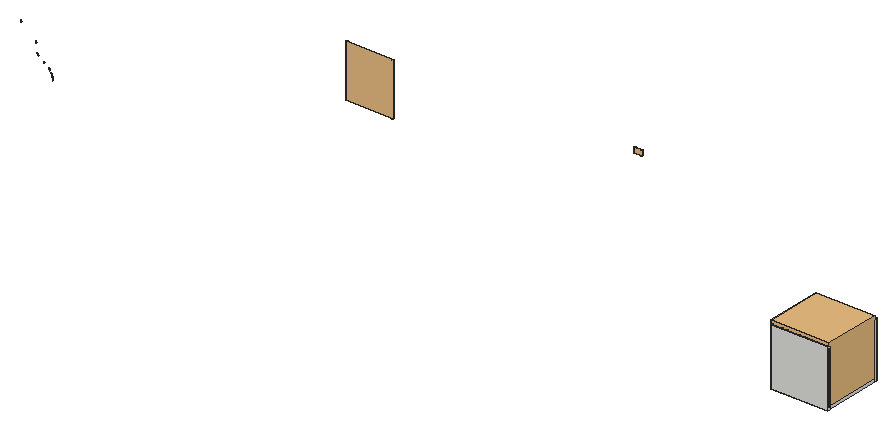
# SketchUp Ruby script. Lengths in inches.
U = 1.inch
M = Sketchup.active_model
def pt(a) = Geom::Point3d.new(a.map { |v| v * U })
def face(e, loops, mat)
  f = e.add_face(loops[0].map { |a| pt(a) })
  loops[1..].each { |l| e.add_face(l.map { |a| pt(a) }).erase! }
  f.material = f.back_material = mat if mat
  f
end
# faces: each face lists its corners as indices into pts; further lists are holes
def faces(e, pts, list, mat = nil) = list.each { |f| face(e, (f[0].is_a?(Array) ? f : [f]).map { |l| l.map { |i| pts[i] } }, mat) }
# xy, xz, yz: faces in a plane at the given z, y or x. An outline is a flat list of corners, or four numbers for a rectangle; further outlines are holes
def ring(l) = l.size == 4 ? [[l[0], l[1]], [l[2], l[1]], [l[2], l[3]], [l[0], l[3]]] : l.each_slice(2).to_a
def flat(e, list, mat, &to3) = list.each { |f| face(e, (f[0].is_a?(Array) ? f : [f]).map { |l| ring(l).map { |u, v| to3.(u, v) } }, mat) }
def xy(e, z, list, mat = nil) = flat(e, list, mat) { |x, y| [x, y, z] }
def xz(e, y, list, mat = nil) = flat(e, list, mat) { |x, z| [x, y, z] }
def yz(e, x, list, mat = nil) = flat(e, list, mat) { |y, z| [x, y, z] }
def lines(e, pts, list) = list.each { |a, b| e.add_line(pt(pts[a]), pt(pts[b])) }
# prism: a flat outline (further loops are holes) pulled along v
def prism(e, loops, v, mat = nil)
  f = face(e, loops, mat); d = Geom::Vector3d.new(v.map { |x| x * U })
  f.pushpull(f.normal.samedirection?(d) ? d.length : -d.length)
end
def box(e, o, s, mat = nil) = prism(e, [[o, [o[0] + s[0], o[1], o[2]], [o[0] + s[0], o[1] + s[1], o[2]], [o[0], o[1] + s[1], o[2]]]], [0, 0, s[2]], mat)
def at(x, y, z, deg = 0) = Geom::Transformation.translation(pt([x, y, z])) * Geom::Transformation.rotation(ORIGIN, Z_AXIS, deg.degrees)
def axes(o, x, y, z) = Geom::Transformation.new([*x, 0, *y, 0, *z, 0, *pt(o).to_a, 1])
def part(name) = M.definitions.add(name)
# library, detail: a bought-in or finely detailed component or shape, given as its bounding box
def library(name, o, s) = part(name).tap { |d| box(d.entities, o, s) }
def detail(e, o, s) = box(e.add_group.entities, o, s)
def put(e, d, t, mat = nil) = e.add_instance(d, t).tap { |i| i.material = mat if mat }
def group(e, t, mat = nil) = e.add_group.tap { |g| g.transformation = t; g.material = mat if mat }.entities
root = M.entities
M.materials.add("Generic\#1").color = [212, 210, 207]
M.materials["Generic\#1"].alpha = 0.64
M.materials.add("[Color_C17]").color = [102, 61, 19]
M.materials.add("[Color_D04]").color = [226, 212, 151]
M.materials.add("[Metal Corrugated Shiny]").color = [126, 126, 126]
M.materials.add("[Translucent Glass Gray]1").color = [186, 186, 186]
M.materials["[Translucent Glass Gray]1"].alpha = 0.5
M.materials.add("[Translucent Glass Gray]2").color = [128, 128, 128]
M.materials["[Translucent Glass Gray]2"].alpha = 0.5
M.materials.add("guide_book_pages_650").color = [228, 220, 176]
M.materials.add("wall texture").color = [149, 150, 148]
c1 = library("bed",[8.45,-2.17,-0.02],[100.66,82.09,31.1])
c2 = part("Grupo\#10")
prism(c2.entities,[[[0.34,1.25,0],[0.5,1.32,0],[0.67,1.34,0],[0.85,1.32,0],[1.01,1.25,0],[1.15,1.15,0],[1.25,1.01,0],[1.32,0.85,0],[1.34,0.67,0],[1.32,0.5,0],[1.25,0.34,0],[1.15,0.2,0],[1.01,0.09,0],[0.85,0.02,0],[0.67,0,0],[0.5,0.02,0],[0.34,0.09,0],[0.2,0.2,0],[0.09,0.34,0],[0.02,0.5,0],[0,0.67,0],[0.02,0.85,0],[0.09,1.01,0],[0.2,1.15,0]]],[0,0,192.91])
c3 = part("Grupo\#1")
put(c3.entities,c2,axes([8.8125,2.875,0.56],[0.0689,0,0],[0,0.06833,0.00887],[0,-0.00887,0.06833]))
put(c3.entities,c2,axes([9.19,1.3125,0.58],[0.06879,0.00048,0.00394],[0,0.0684,-0.00828],[-0.00397,0.00826,0.06829]))
put(c3.entities,c2,axes([8.9,0.97,1.35],[0.0689,0,0],[0,0.06788,-0.01185],[0,0.01185,0.06788]))
put(c3.entities,c2,axes([9.375,1.96,0.37],[0.06868,0,0.00553],[0,0.0689,0],[-0.00553,0,0.06868]))
put(c3.entities,c2,axes([7.76,2.02,1.22],[0.06788,0,-0.01185],[0,0.0689,0],[0.01185,0,0.06788]))
g1 = group(c3.entities,at(6.375,-0.82,0))
detail(g1,[0,0,0],[4.31,4.31,6.9375])
c4 = part("Difusor aromático\#1")
put(c4.entities,c3,at(-1.02,1.61,-0.92),"[Translucent Glass Gray]2")
c5 = part("Book\#1")
xy(c5.entities,0,[[0,0,199.1,147.6]],"[Color_C17]")
xy(c5.entities,1.64,[[0,0,3.4,147.6],[195.7,0,199.1,147.6]],"[Color_C17]")
xz(c5.entities,0,[[0,0,199.1,1.64]],"[Color_C17]")
xz(c5.entities,0,[[3.4,1.64,195.7,1.64,193.74,6.22,190.64,6.23,187.55,6.32,184.47,6.49,181.39,6.75,178.34,7.1,175.31,7.53,172.3,8.04,166.83,9.33,161.3,10.51,155.73,11.57,150.11,12.51,144.46,13.33,138.77,14.04,133.05,14.62,127.79,14.85,122.53,14.58,117.37,13.8125,112.4,12.57,107.72,10.87,103.41,8.74,99.55,6.22,95.6875,9.67,91.38,12.58,86.7,14.92,81.73,16.62,76.57,17.67,71.3125,18.04,66.05,17.73,60.33,16.93,54.64,15.96,48.99,14.84,43.37,13.55,37.8,12.1,32.27,10.48,26.8,8.71,23.79,8.01,20.76,7.42,17.71,6.95,14.64,6.59,11.55,6.35,8.46,6.23,5.37,6.22]],"[Color_D04]")
xz(c5.entities,147.6,[[0,0,199.1,1.64]],"[Color_C17]")
xz(c5.entities,147.6,[[3.4,1.64,5.37,6.22,8.46,6.23,11.55,6.35,14.64,6.59,17.71,6.95,20.76,7.42,23.79,8.01,26.8,8.71,32.27,10.48,37.8,12.1,43.37,13.55,48.99,14.84,54.64,15.96,60.33,16.93,66.05,17.73,71.3125,18.04,76.57,17.67,81.73,16.62,86.7,14.92,91.38,12.58,95.6875,9.67,99.55,6.22,103.41,8.74,107.72,10.87,112.4,12.57,117.37,13.8125,122.53,14.58,127.79,14.85,133.05,14.62,138.77,14.04,144.46,13.33,150.11,12.51,155.73,11.57,161.3,10.51,166.83,9.33,172.3,8.04,175.31,7.53,178.34,7.1,181.39,6.75,184.47,6.49,187.55,6.32,190.64,6.23,193.74,6.22,195.7,1.64]],"[Color_D04]")
yz(c5.entities,0,[[0,0,147.6,1.64]],"[Color_C17]")
yz(c5.entities,199.1,[[0,0,147.6,1.64]],"[Color_C17]")
p = [[3.4,0,1.64],[5.37,0,6.22],[5.37,147.6,6.22],[3.4,147.6,1.64],[193.74,0,6.22],[195.7,0,1.64],
  [195.7,147.6,1.64],[193.74,147.6,6.22],[8.46,0,6.23],[8.46,147.6,6.23],[11.55,0,6.35],[11.55,147.6,6.35],
  [95.6875,0,9.67],[99.55,0,6.22],[99.55,147.6,6.22],[95.6875,147.6,9.67],[103.41,0,8.74],[103.41,147.6,8.74],
  [187.55,0,6.32],[190.64,0,6.23],[190.64,147.6,6.23],[187.55,147.6,6.32],[184.47,0,6.49],[184.47,147.6,6.49],
  [14.64,0,6.59],[14.64,147.6,6.59],[181.39,0,6.75],[181.39,147.6,6.75],[17.71,0,6.95],[17.71,147.6,6.95],
  [178.34,0,7.1],[178.34,147.6,7.1],[20.76,0,7.42],[20.76,147.6,7.42],[175.31,0,7.53],[175.31,147.6,7.53],
  [23.79,0,8.01],[23.79,147.6,8.01],[172.3,0,8.04],[172.3,147.6,8.04],[26.8,0,8.71],[26.8,147.6,8.71],
  [166.83,0,9.33],[166.83,147.6,9.33],[32.27,0,10.48],[32.27,147.6,10.48],[107.72,0,10.87],[107.72,147.6,10.87],
  [161.3,0,10.51],[161.3,147.6,10.51],[91.38,0,12.58],[91.38,147.6,12.58],[37.8,0,12.1],[37.8,147.6,12.1],
  [155.73,0,11.57],[155.73,147.6,11.57],[112.4,0,12.57],[112.4,147.6,12.57],[150.11,0,12.51],[150.11,147.6,12.51],
  [43.37,0,13.55],[43.37,147.6,13.55],[144.46,0,13.33],[144.46,147.6,13.33],[86.7,0,14.92],[86.7,147.6,14.92],
  [117.37,0,13.8125],[117.37,147.6,13.8125],[138.77,0,14.04],[138.77,147.6,14.04],[48.99,0,14.84],[48.99,147.6,14.84],
  [122.53,0,14.58],[122.53,147.6,14.58],[133.05,0,14.62],[133.05,147.6,14.62],[127.79,0,14.85],[127.79,147.6,14.85],
  [54.64,0,15.96],[54.64,147.6,15.96],[81.73,0,16.62],[81.73,147.6,16.62],[60.33,0,16.93],[60.33,147.6,16.93],
  [76.57,0,17.67],[76.57,147.6,17.67],[66.05,0,17.73],[66.05,147.6,17.73],[71.3125,0,18.04],[71.3125,147.6,18.04]]
faces(c5.entities,p,[[0,1,2,3],[4,5,6,7],[1,8,9,2],[8,10,11,9],[12,13,14,15],[13,16,17,14],[18,19,20,21],[19,4,7,20],
  [22,18,21,23],[10,24,25,11],[26,22,23,27],[24,28,29,25],[30,26,27,31],[28,32,33,29],[34,30,31,35],[32,36,37,33],
  [38,34,35,39],[36,40,41,37],[42,38,39,43],[40,44,45,41],[16,46,47,17],[48,42,43,49],[50,12,15,51],[44,52,53,45],
  [54,48,49,55],[46,56,57,47],[58,54,55,59],[52,60,61,53],[62,58,59,63],[64,50,51,65],[56,66,67,57],[68,62,63,69],
  [60,70,71,61],[66,72,73,67],[74,68,69,75],[72,76,77,73],[76,74,75,77],[70,78,79,71],[80,64,65,81],[78,82,83,79],
  [84,80,81,85],[82,86,87,83],[86,88,89,87],[88,84,85,89]],"guide_book_pages_650")
c6 = library("Glasses\#1",[0,0,0],[79.32,78.74,17.6])
c7 = library("Group\#5",[0,0,0],[21.15,0.01,14.26])
c8 = library("Group\#8",[0,0,0],[102.14,0.5,111.36])
c9 = library("Group\#17",[0,0,0],[28.72,28.74,77])
c10 = part("Square rod")
xy(c10.entities,-0.04,[[0.04,0.04,0.36,0.36]])
xy(c10.entities,0,[[[0,0,0.39,0.39],[0.04,0.04,0.36,0.36]]])
xy(c10.entities,19.69,[[0,0,0.39,0.39]])
xz(c10.entities,0,[[0,0,0.39,19.69]])
xz(c10.entities,0.04,[[0.04,-0.04,0.36,0]])
xz(c10.entities,0.36,[[0.04,-0.04,0.36,0]])
xz(c10.entities,0.39,[[0,0,0.39,19.69]])
yz(c10.entities,0,[[0,0,0.39,19.69]])
yz(c10.entities,0.04,[[0.04,-0.04,0.36,0]])
yz(c10.entities,0.36,[[0.04,-0.04,0.36,0]])
yz(c10.entities,0.39,[[0,0,0.39,19.69]])
c11 = part("Group\#626")
box(c11.entities,[0,0,0],[0.39,18.9,0.39])
c12 = part("Group\#630")
box(c12.entities,[0,0,0],[18.9,0.39,0.39])
c13 = library("Group\#635",[0,0,0],[3.14,3.14,10.11])
c14 = library("Group\#634",[0,0,0],[7.05,7.05,10.1])
c15 = library("Group\#633",[0,0,0],[47.27,36.83,57.22])
c16 = library("Group\#632",[0,0,0],[63.43,39.67,4.76])
c17 = library("Group\#639",[0,0,0],[29.35,22.46,29.82])
xz(root,68.94,[[68.26,0,67.897,2.998,67.579,4.474,67.288,5.822,68.136,6.149,68.144,6.152,68.135,6.15,67.632,6.075,67.231,6.044,66.358,8.824,67.116,7.869,68.125,6.184,67.294,8.831,66.128,11.616,64.712,14.283,63.056,16.809,61.45,18.827,61.176,19.172,59.596,20.821,60.055,20.229,61.45,18.827,63.056,16.809,64.712,14.283,66.128,11.616,67.294,8.831,68.125,6.184,68.135,6.15,68.136,6.149,68.198,5.95,68.516,4.474,68.835,2.998,69.197,0],[61.45,18.827,60.055,20.229,59.596,20.821,61.176,19.172],[50.479,26.777,50.392,26.818,50.718,27.105],[50.718,27.105,49.015,27.904,48.649,28.08,48.921,27.989],[38.749,35.828,38.683,35.912,38.746,35.834],
  [38.683,35.912,38.208,36.506,38.149,36.599],[38.149,36.599,37.535,37.389,36.522,39.088,35.726,40.898,35.718,40.926,36.714,38.871],[32.979,59.945,32.975,59.997,32.405,62.383,32.196,62.884,32.966,61.774,33.882,59.994,33.365,59.95],[1.729,87.284,1.661,87.435,0.638,89.676,0,90.727,0.145,90.599,1.465,89.094,2.576,87.429,2.068,87.327]])
# 1073 loose lines left out
detail(root,[485.1,319.58,0.05],[101.58,0.05,110.82])
detail(root,[1634.04,3.5,0],[124,120,126])
put(root,c1,axes([1701.17,19.22,6.01],[0,0.79,0],[-0.79,0,0],[0,0,0.79]))
put(root,c4,axes([1650.16,104.91,26],[0.29449,-0.03616,0],[0.03616,0.29449,0],[0,0,0.2967]))
put(root,c5,axes([1659.12,112.75,21.39],[0.01748,-0.03819,0],[0.03819,0.01748,0],[0,0,0.042]))
put(root,c6,axes([1660.36,111.62,22.1875],[0.01391,-0.0393,-0.00511],[0.03953,0.01414,-0.00114],[0.00279,-0.00443,0.04167]))
g2 = group(root,at(1758.04,3.5,0,90))
xy(g2,0,[[0,0,120,120]])
xy(g2,6,[[0,0,120,120]],"Generic\#1")
xz(g2,0,[[0,0,120,6]])
xz(g2,120,[[0,0,120,6]])
yz(g2,0,[[0,0,120,6]])
yz(g2,120,[[0,0,120,6]])
g3 = group(root,at(1758.04,127.5,0,180))
xy(g3,0,[[0,0,120,4]])
xy(g3,120,[[0,0,120,4]])
xz(g3,0,[[0,0,120,120]])
xz(g3,4,[[0,0,120,120]],"wall texture")
yz(g3,0,[[0,0,4,120]])
yz(g3,120,[[0,0,4,120]])
put(root,c7,axes([968.64,475.68,1.17],[0.86,0,0],[0,0.86,0],[0,0,0.86]))
g4 = group(root,at(1638.04,0,6))
xy(g4,-6,[[0,0,120,4]])
xy(g4,114,[[0,0,120,4]])
xz(g4,0,[[0,-6,120,114]])
xz(g4,4,[[118.939,5.841,118.938,5.843,118.947,5.844]])
yz(g4,0,[[0,-6,4,114]])
yz(g4,120,[[0,-6,4,114]])
# 341 loose lines left out
detail(g4,[0.02,2,0.03],[120,1.5,114])
put(g4,c8,axes([17.86,3.6875,0],[1,0,0],[0,1,0],[0,0,0.95]))
put(root,c9,axes([1649.82,10.52,79.19],[0.53,0,0],[0,0.53,0],[0,0,0.53]))
put(root,c9,axes([1644.52,108.27,79.19],[0.53,0,0],[0,0.53,0],[0,0,0.53]))
g5 = group(root,at(1640.91,8.49,21.39))
xy(g5,0,[[[0,0,19.291,18.898],[0.394,0.394,18.898,18.504]],[0.394,0.394,18.898,18.504]])
xy(g5,1.581,[[0,0,18.898,0.197],[0,18.701,18.898,18.898]])
xy(g5,2.172,[[0,0,18.898,0.197],[0,18.701,18.898,18.898]])
xy(g5,3.917,[[0,0,19.291,0,19.291,7.874,18.898,7.874,18.898,0.394,0.394,0.394,0.394,18.504,18.898,18.504,18.898,11.024,19.291,11.024,19.291,18.898,0,18.898]])
xz(g5,0,[[0,0,19.291,0,19.291,3.917,0,3.917,0,2.172,18.898,2.172,18.898,1.581,0,1.581]])
xz(g5,0.197,[[0,1.581,18.898,2.172]])
xz(g5,0.394,[[0.394,0,18.898,3.917]])
xz(g5,18.504,[[0.394,0,18.898,3.917]])
xz(g5,18.701,[[0,1.581,18.898,2.172]])
xz(g5,18.898,[[0,0,0,1.581,18.898,1.581,18.898,2.172,0,2.172,0,3.917,19.291,3.917,19.291,0]])
yz(g5,0,[[0,0,0,1.581,0.197,1.581,0.197,2.172,0,2.172,0,3.917,18.898,3.917,18.898,2.172,18.701,2.172,18.701,1.581,18.898,1.581,18.898,0]])
yz(g5,0.394,[[0.394,0,18.504,3.917]])
yz(g5,18.898,[[0.394,0,0.394,3.917,7.874,3.917,7.874,3.937,7.91,3.937,7.91,3.25,7.913,3.231,7.915,3.224,7.918,3.217,7.923,3.21,7.928,3.204,7.935,3.199,7.941,3.194,7.949,3.19,7.955,3.188,7.975,3.186,10.934,3.187,10.941,3.188,10.949,3.19,10.956,3.194,10.963,3.199,10.969,3.204,10.975,3.21,10.983,3.224,10.985,3.232,10.987,3.239,10.988,3.937,11.024,3.937,11.024,3.917,18.504,3.917,18.504,0],[0,1.581,0.197,2.172],[18.701,1.581,18.898,2.172]])
yz(g5,19.291,[[0,0,18.898,0,18.898,3.917,11.024,3.917,11.023,3.235,11.02,3.223,11.016,3.21,11.01,3.199,11.003,3.188,10.995,3.178,10.985,3.17,10.974,3.163,10.963,3.157,10.951,3.153,10.938,3.15,7.972,3.15,7.947,3.153,7.935,3.157,7.923,3.163,7.913,3.17,7.903,3.178,7.894,3.188,7.887,3.199,7.882,3.21,7.877,3.223,7.874,3.248,7.874,3.917,0,3.917]])
g6 = group(g5,at(18.9,7.875,3.15),"[Metal Corrugated Shiny]")
detail(g6,[0,0,0],[0.43,3.15,0.79])
g7 = group(root,at(1640.52,8.1,6),"[Metal Corrugated Shiny]")
p = [[19.69,0.39,0.04],[19.69,0.39,0.83],[19.69,0.39,19.33],[19.69,0.39,17.36],[19.69,0.39,15.39]]
lines(g7,p,[[0,1],[2,3],[3,4]])
put(g7,c10,at(19.29,19.29,0.04))
put(g7,c10,at(0,0,0.04))
put(g7,c10,at(19.29,0,0.04))
put(g7,c10,at(0,19.29,0.04))
put(g7,c11,at(0,0.39,17.17))
g8 = group(g7,at(0,0,19.33),"[Metal Corrugated Shiny]")
prism(g8,[[[19.29,0,0],[0.39,0,0],[0.39,0.39,0],[0,0.39,0],[0,19.29,0],[0.39,19.29,0],[0.39,19.69,0],[19.29,19.69,0],[19.29,19.29,0],[19.69,19.29,0],[19.69,0.39,0],[19.29,0.39,0]]],[0,0,0.39])
g9 = group(g7,at(0.39,19.29,17.17))
box(g9,[0,-0.2,0],[18.9,0.59,0.39])
g10 = group(g7,at(0.39,0,17.17))
box(g10,[0,0,0],[18.9,0.59,0.39])
put(g7,c12,at(0.39,19.29,0.83))
put(g7,c11,at(0,0.39,0.83))
put(g7,c12,at(0.39,0,0.83))
put(g7,c11,at(19.29,0.39,0.83))
put(root,c13,axes([1654.42,108.88,25.77],[-0.29784,-0.40546,0],[0.40546,-0.29784,0],[0,0,0.5031]))
g11 = group(root,at(1647.45,103.85,25.72),"[Translucent Glass Gray]1")
xy(g11,0,[[[10.08,-1.24,0,0,0.93,7.5625,11.01,6.32],[9.86,-0.95,10.73,6.1,1.15,7.28,0.28,0.22]],[9.86,-0.95,0.28,0.22,1.15,7.28,10.73,6.1]])
xy(g11,0.51,[[10.42,1.53,10.67,3.55,10.42,3.58,10.17,1.57],[0.59,2.74,0.84,4.76,0.59,4.79,0.34,2.77]])
xy(g11,0.89,[[10.42,1.53,10.17,1.57,10.42,3.58,10.67,3.55],[0.59,2.74,0.34,2.77,0.59,4.79,0.84,4.76]])
xy(g11,1.02,[[[10.08,-1.24,11.01,6.32,0.93,7.5625,0,0],[9.86,-0.95,0.28,0.22,1.15,7.28,10.73,6.1]]])
p = [[0,0,0],[10.08,-1.24,0],[10.08,-1.24,1.02],[0,0,1.02],[11.01,6.32,0],[11.01,6.32,1.02],
  [10.42,1.53,0.89],[10.67,3.55,0.89],[10.67,3.55,0.51],[10.42,1.53,0.51],[9.86,-0.95,0],[0.28,0.22,0],
  [0.28,0.22,1.02],[9.86,-0.95,1.02],[10.73,6.1,0],[10.73,6.1,1.02],[10.17,1.57,0.89],[10.17,1.57,0.51],
  [10.42,3.58,0.51],[10.42,3.58,0.89],[0.93,7.5625,1.02],[0.93,7.5625,0],[0.59,4.79,0.89],[0.34,2.77,0.89],
  [0.34,2.77,0.51],[0.59,4.79,0.51],[1.15,7.28,0],[1.15,7.28,1.02],[0.59,2.74,0.89],[0.84,4.76,0.89],
  [0.84,4.76,0.51],[0.59,2.74,0.51]]
faces(g11,p,[[0,1,2,3],[[1,4,5,2],[6,7,8,9]],[10,11,12,13],[[14,10,13,15],[16,17,18,19]],[[3,20,21,0],[22,23,24,25]],[[11,26,27,12],[28,29,30,31]],[26,14,15,27],[4,21,20,5],
  [17,16,6,9],[24,23,28,31],[19,18,8,7],[22,25,30,29]])
put(root,c14,at(1643.09,11.19,25.72))
put(root,c15,axes([1647.72,10.5625,25.72],[0.165,0.28579,0],[-0.28579,0.165,0],[0,0,0.33]))
put(root,c16,axes([1654.98,15.43,25.72],[0.05391,0.01087,0],[-0.01087,0.05391,0],[0,0,0.055]))
put(root,c17,at(1642.98,95.99,6,6.5))
